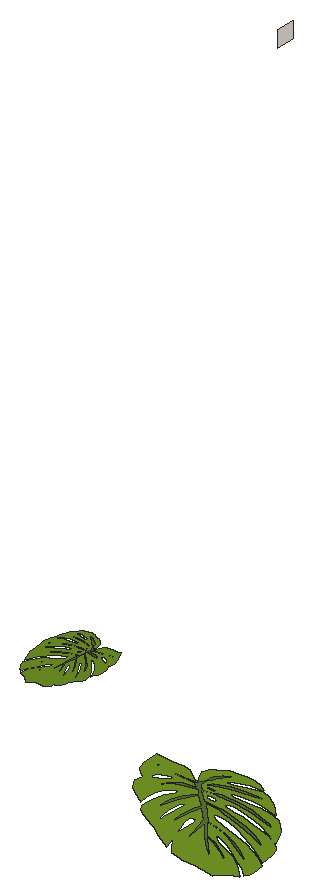
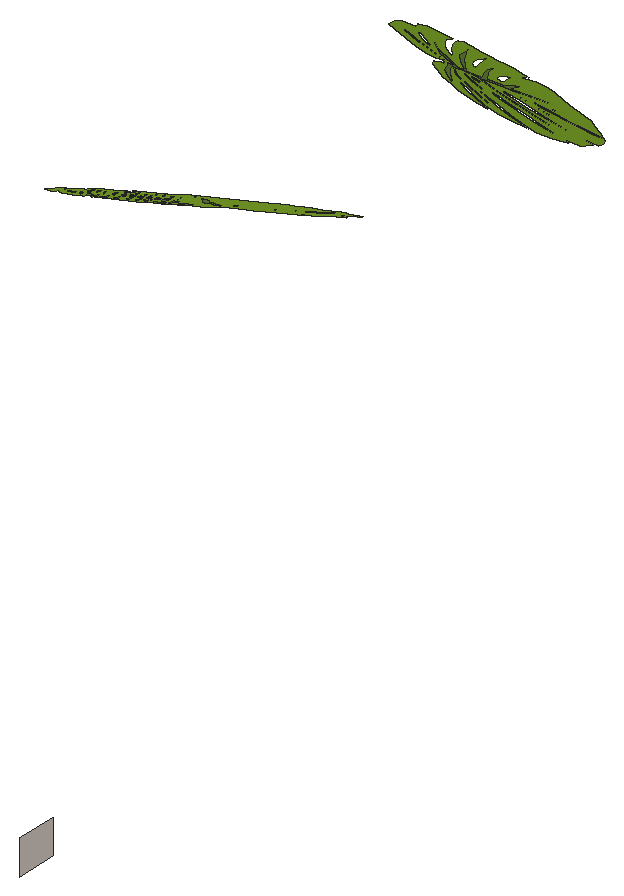
# SketchUp Ruby script. Lengths in inches.
U = 1.inch
M = Sketchup.active_model
def pt(a) = Geom::Point3d.new(a.map { |v| v * U })
def face(e, loops, mat)
  f = e.add_face(loops[0].map { |a| pt(a) })
  loops[1..].each { |l| e.add_face(l.map { |a| pt(a) }).erase! }
  f.material = f.back_material = mat if mat
  f
end
# faces: each face lists its corners as indices into pts; further lists are holes
def faces(e, pts, list, mat = nil) = list.each { |f| face(e, (f[0].is_a?(Array) ? f : [f]).map { |l| l.map { |i| pts[i] } }, mat) }
# xy, xz, yz: faces in a plane at the given z, y or x. An outline is a flat list of corners, or four numbers for a rectangle; further outlines are holes
def ring(l) = l.size == 4 ? [[l[0], l[1]], [l[2], l[1]], [l[2], l[3]], [l[0], l[3]]] : l.each_slice(2).to_a
def flat(e, list, mat, &to3) = list.each { |f| face(e, (f[0].is_a?(Array) ? f : [f]).map { |l| ring(l).map { |u, v| to3.(u, v) } }, mat) }
def xy(e, z, list, mat = nil) = flat(e, list, mat) { |x, y| [x, y, z] }
def xz(e, y, list, mat = nil) = flat(e, list, mat) { |x, z| [x, y, z] }
def yz(e, x, list, mat = nil) = flat(e, list, mat) { |y, z| [x, y, z] }
def lines(e, pts, list) = list.each { |a, b| e.add_line(pt(pts[a]), pt(pts[b])) }
# prism: a flat outline (further loops are holes) pulled along v
def prism(e, loops, v, mat = nil)
  f = face(e, loops, mat); d = Geom::Vector3d.new(v.map { |x| x * U })
  f.pushpull(f.normal.samedirection?(d) ? d.length : -d.length)
end
def box(e, o, s, mat = nil) = prism(e, [[o, [o[0] + s[0], o[1], o[2]], [o[0] + s[0], o[1] + s[1], o[2]], [o[0], o[1] + s[1], o[2]]]], [0, 0, s[2]], mat)
def at(x, y, z, deg = 0) = Geom::Transformation.translation(pt([x, y, z])) * Geom::Transformation.rotation(ORIGIN, Z_AXIS, deg.degrees)
def axes(o, x, y, z) = Geom::Transformation.new([*x, 0, *y, 0, *z, 0, *pt(o).to_a, 1])
def part(name) = M.definitions.add(name)
# library, detail: a bought-in or finely detailed component or shape, given as its bounding box
def library(name, o, s) = part(name).tap { |d| box(d.entities, o, s) }
def detail(e, o, s) = box(e.add_group.entities, o, s)
def put(e, d, t, mat = nil) = e.add_instance(d, t).tap { |i| i.material = mat if mat }
def group(e, t, mat = nil) = e.add_group.tap { |g| g.transformation = t; g.material = mat if mat }.entities
root = M.entities
M.materials.add("[0009_Linen]").color = [250, 240, 230]
M.materials.add("[0059_DarkOliveGreen]").color = [85, 107, 47]
M.materials.add("[0061_OliveDrab]").color = [107, 142, 35]
yz(root,328.15,[[300.43,52.25,304.24,55.45]],"[0009_Linen]")
p = [[413.85,165,15.87],[412.66,164.86,16.11],[411.93,162.875,15.41],[411.97,161.6875,14.86],[412.59,161,14.39],[413.3,160.66,14.0625],
  [412.59,159.58,13.75],[413.01,158.58,13.2],[413.77,158.02,12.75],[415.21,157.53,12.16],[415.68,157.3,11.9375],[415.78,158.5,12.45],
  [416.43,159.72,12.83],[417.45,160.89,13.1],[418.7,161.74,13.15],[419.1,161.9,13.125],[419.24,161.84,13.06],[419.08,161.55,12.97],
  [417.8,160.16,12.68],[416.96,158.93,12.34],[416.26,157.61,11.93],[416.06,156.91,11.67],[416.37,156.3,11.3125],[417.08,155.97,10.98],
  [418.26,155.62,10.52],[419.35,155.32,10.11],[419.91,155.17,9.9],[420.84,154.625,9.41],[421.91,154.24,8.96],[423.01,154.01,8.57],
  [423.59,153.85,8.36],[423.5,154.52,8.68],[423.4,155.52,9.16],[424.51,153.73,8.0625],[424.8125,153.51,7.89],[425.83,153.45,7.6],
  [426.85,153.39,7.31],[429.17,153.85,6.92],[432.48,154.08,6.17],[433.8125,155.1875,6.32],[435.15,155.97,6.33],[436.01,156.4,6.3],
  [434.34,157.54,7.24],[433.04,158.16,7.86],[431.18,158.59,8.53],[429.86,158.85,8.99],[429.22,159.16,9.29],[428.7,159.41,9.53],
  [428.7,159.58,9.61],[429.05,159.63,9.54],[430.09,159.5,9.22],[430.97,159.28,8.89],[432.78,158.59,8.12],[434.29,157.96,7.44],
  [435.26,157.62,7.04],[435.89,157.21,6.7],[436.35,156.78,6.38],[437.04,157.45,6.51],[437.36,158.02,6.68],[437.53,158.54,6.87],
  [437.6,158.94,7.03],[437.78,159.42,7.2],[436.29,160.31,7.98],[434.875,160.78,8.56],[433.64,161,8.98],[431.33,161.24,9.68],
  [429.57,161.3125,10.16],[428.09,161.42,10.59],[426.98,161.5625,10.94],[426.45,161.81,11.19],[426.42,162.15,11.35],[427.25,162.3,11.2],
  [428.39,162.39,10.95],[430.39,162.22,10.36],[432.54,161.79,9.62],[434.92,161.12,8.7],[437.6,160.09,7.55],[437.9,161.81,8.24],
  [437.9375,162.83,8.69],[437.51,163.27,9],[436.53,163.74,9.46],[435.33,164.01,9.89],[433.71,164.12,10.36],[432.33,164.19,10.75],
  [430.29,164.28,11.3125],[428.78,164.22,11.67],[427.6,164.17,11.95],[427.03,164.11,12.07],[426.7,164.26,12.23],[427.05,164.5,12.25],
  [427.92,164.81,12.16],[429.29,164.95,11.87],[432.06,164.83,11.1],[433.6875,164.64,10.6],[435.14,164.38,10.11],[435.81,164.14,9.83],
  [437.14,163.74,9.31],[437.19,164.03,9.42],[436.87,165.02,9.95],[436.52,165.9,10.4375],[435.17,166.9,11.23],[433.76,167.09,11.68],
  [431.5,166.95,12.2],[429.51,166.53,12.52],[427.69,166.23,12.85],[426.9,166.07,12.99],[426.45,166.1,13.12],[426.5,166.28,13.18],
  [427.42,166.65,13.11],[429.64,167.18,12.78],[431.45,167.33,12.38],[434.32,167.32,11.64],[432.88,168.51,12.54],[431.41,169.13,13.2],
  [430.1875,169.24,13.5625],[429.55,169.04,13.64],[427.65,168.38,13.83],[426.23,167.77,13.92],[425.12,167.39,14.04],[424.68,167.35,14.13],
  [424.54,167.51,14.24],[424.78,167.68,14.25],[426.56,168.48,14.16],[427.99,168.93,13.99],[429.26,169.23,13.8],[430.22,169.43,13.64],
  [429.04,169.87,14.14],[427.93,170,14.49],[426.5,169.8125,14.77],[425.16,169.43,14.94],[423.79,169.16,15.17],[423.08,168.68,15.14],
  [421.9,168.09,15.18],[420.89,167.41,15.14],[420.4,166.5,14.85],[420.55,165.56,14.39],[420.89,165.01,14.06],[420.2,164.81,14.14],
  [419.625,165.26,14.5],[418.65,165.72,14.95],[417.39,165.69,15.27],[415.54,165.35,15.59],[417.35,163.83,14.44],[413.875,163.56,15.21],
  [416.11,163.94,14.8125],[420.77,164.75,13.97],[421.34,165.45,14.14],[422.24,166.95,14.58],[423.42,167.88,14.7],[424.45,168.43,14.68],
  [422.86,166.86,14.38],[421.93,165.56,14.04],[421.63,164.83,13.79],[422.94,165.99,13.97],[425.51,167.09,13.8],[427.57,167.66,13.53],
  [429.69,168.11,13.1875],[430.76,168.25,12.97],[427.48,167.34,13.41],[425.53,166.7,13.625],[423.38,165.83,13.79],[422.26,165.08,13.74],
  [421.8,164.66,13.66],[421.92,164.39,13.52],[422.27,164.34,13.4],[423.22,164.59,13.27],[424.17,165,13.21],[425.3,165.27,13.04],
  [428.57,165.79,12.43],[430.65,165.95,11.97],[432.61,165.8,11.4],[434.19,165.7,10.95],[434.79,165.42,10.66],[431.74,165.625,11.54],
  [430.01,165.56,11.96],[427.28,165.27,12.53],[424.87,164.77,12.93],[422.24,164.1,13.3],[423.61,163.03,12.47],[425.64,163.29,12.06],
  [427.5625,163.49,11.66],[431.54,163.29,10.55],[433.51,162.92,9.87],[434.83,162.59,9.39],[435.44,162.3,9.1],[433.58,162.65,9.73],
  [430.51,162.96,10.66],[426.58,163.0625,11.72],[424.22,162.74,12.18],[426.33,160.69,10.72],[427.91,160.84,10.38],[429.85,160.64,9.79],
  [431.71,160.18,9.11],[433.11,159.7,8.53],[434.65,158.97,7.81],[431.46,160,9.09],[429.62,160.42,9.75],[427.9,160.56,10.26],
  [426.35,160.45,10.61],[427.6875,158.86,9.55],[429.39,158.57,8.98],[430.92,158.08,8.37],[432.17,157.48,7.78],[432.72,156.9,7.375],
  [430.625,157.9,8.36],[429.06,158.3,8.94],[427.8,158.53,9.37],[429.09,157.29,8.48],[429.77,156.63,8.01],[430.74,155.78,7.38],
  [430.57,155.89,7.48],[428.69,157.14,8.52],[427.2,158.4,9.47],[426.0625,159.92,10.44],[425.3,156.34,9.03],[425.31,160.42,10.86],
  [423.96,161.63,11.75],[422.75,159.88,11.28],[421.51,157.05,10.33],[421.95,159.13,11.15],[422.87,161.0625,11.78],[423.61,162.08,12.04],
  [422.29,163.09,12.83],[420.16,160.89,12.4],[418.05,157.68,11.5],[418.92,160.25,12.43],[420.4,161.95,12.8125],[422.03,163.4,13.04],
  [421.59,163.82,13.34],[419.95,163.24,13.51],[417.77,162.48,13.73],[415.57,160.74,13.51],[417.07,162.3,13.83],[418.79,163.47,13.9],
  [420.73,163.92,13.61],[421.05,164.13,13.62],[420.41,164.43,13.92],[420.16,159.31,11.6875],[420.89,160.49,12.03],[421.27,160.78,12.0625],
  [421.54,160.85,12.02],[421.65,160.71,11.93],[421.43,160.24,11.78],[420.9,159.11,11.41],[420.33,157.87,11],[419.89,156.5625,10.53],
  [419.66,155.95,10.31],[419.72,157.81,11.125],[423.55,159.45,10.88],[423.89,159.875,10.98],[424.29,159.9,10.89],[424.5,159.71,10.75],
  [424.54,159.3,10.56],[424.4,158.97,10.44],[423.89,157.66,9.99],[423.4,156.44,9.57],[423.33,158.3,10.42],[414.96,162.42,14.42],
  [415.93,162.94,14.4],[416.79,163.24,14.32],[417.25,163.21,14.1875],[417.4,163.07,14.09],[415.97,162.18,14.06],[414.7,161.48,14.07],
  [414.33,161.35,14.1],[414.36,161.85,14.32],[423.95,164.2,12.91],[424.6875,164.24,12.74],[425.24,164.08,12.52],[425.1875,163.86,12.4375],
  [424.48,163.625,12.51],[423.63,163.68,12.75],[423.36,163.9375,12.94],[422.67,165.07,13.63],[423.43,165.26,13.51],[424,165.26,13.37],
  [423.98,165.04,13.27],[423.15,164.84,13.4],[422.55,164.82,13.55],[406.4375,162.9,32.91],[407.23,162.8,33.07],[407.7,161.5,32.61],
  [407.68,160.71,32.25],[407.27,160.26,31.94],[406.81,160.03,31.72],[407.27,159.32,31.52],[406.99,158.66,31.15],[406.49,158.29,30.86],
  [405.54,157.96,30.47],[405.23,157.82,30.32],[405.17,158.6,30.66],[404.74,159.41,30.91],[404.07,160.19,31.08],[403.24,160.75,31.12],
  [402.97,160.85,31.1],[402.88,160.81,31.06],[402.99,160.62,31],[403.84,159.7,30.81],[404.39,158.89,30.59],[404.85,158.02,30.3125],
  [404.98,157.56,30.14],[404.78,157.16,29.91],[404.31,156.9375,29.69],[403.53,156.7,29.38],[402.81,156.51,29.11],[402.44,156.41,28.97],
  [401.83,156.05,28.65],[401.12,155.79,28.36],[400.4,155.64,28.1],[400.01,155.54,27.96],[400.07,155.98,28.17],[400.14,156.64,28.48],
  [399.41,155.46,27.76],[399.2,155.32,27.65],[398.53,155.27,27.46],[397.86,155.23,27.27],[396.33,155.54,27.01],[394.14,155.6875,26.51],
  [393.26,156.42,26.62],[392.38,156.93,26.62],[391.82,157.22,26.6],[392.91,157.97,27.22],[393.77,158.38,27.625],[395,158.66,28.07],
  [395.87,158.84,28.37],[396.29,159.04,28.57],[396.64,159.21,28.73],[396.64,159.32,28.78],[396.41,159.35,28.74],[395.72,159.27,28.53],
  [395.14,159.125,28.3125],[393.95,158.67,27.8],[392.95,158.25,27.35],[392.3125,158.02,27.09],[391.9,157.75,26.86],[391.59,157.47,26.65],
  [391.14,157.91,26.74],[390.93,158.29,26.85],[390.8125,158.63,26.98],[390.76,158.9,27.08],[390.65,159.22,27.2],[391.63,159.8,27.71],
  [392.5625,160.11,28.09],[393.38,160.25,28.36],[394.9,160.42,28.83],[396.0625,160.46,29.15],[397.04,160.53,29.43],[397.78,160.63,29.66],
  [398.125,160.79,29.83],[398.15,161.02,29.93],[397.6,161.11,29.84],[396.84,161.17,29.67],[395.52,161.06,29.28],[394.11,160.78,28.79],
  [392.54,160.33,28.18],[390.77,159.65,27.42],[390.57,160.79,27.88],[390.54,161.46,28.18],[390.82,161.76,28.38],[391.47,162.07,28.6875],
  [392.26,162.24,28.97],[393.33,162.3125,29.28],[394.24,162.36,29.53],[395.59,162.42,29.91],[396.59,162.38,30.15],[397.36,162.35,30.33],
  [397.74,162.31,30.41],[397.96,162.41,30.51],[397.73,162.57,30.52],[397.16,162.77,30.46],[396.25,162.87,30.28],[394.42,162.78,29.77],
  [393.35,162.66,29.43],[392.39,162.49,29.11],[391.95,162.33,28.93],[391.07,162.07,28.58],[391.03,162.25,28.66],[391.25,162.91,29.01],
  [391.48,163.49,29.33],[392.37,164.15,29.85],[393.3,164.28,30.15],[394.79,164.18,30.49],[396.1,163.91,30.71],[397.3,163.71,30.92],
  [397.83,163.6,31.01],[398.125,163.62,31.1],[398.09,163.74,31.14],[397.48,163.99,31.1],[396.02,164.33,30.875],[394.83,164.43,30.61],
  [392.93,164.43,30.12],[393.88,165.21,30.72],[394.85,165.625,31.15],[395.66,165.69,31.39],[396.08,165.5625,31.44],[397.33,165.125,31.57],
  [398.27,164.73,31.63],[399,164.47,31.71],[399.29,164.45,31.77],[399.39,164.55,31.84],[399.23,164.66,31.85],[398.05,165.19,31.78],
  [397.11,165.49,31.68],[396.27,165.6875,31.55],[395.63,165.82,31.44],[396.42,166.11,31.77],[397.15,166.2,32],[398.09,166.07,32.1875],
  [398.98,165.82,32.3],[399.88,165.64,32.46],[400.35,165.32,32.43],[401.13,164.9375,32.46],[401.8,164.49,32.43],[402.11,163.89,32.24],
  [402.02,163.27,31.94],[401.79,162.9,31.72],[402.25,162.77,31.78],[402.63,163.07,32.01],[403.27,163.375,32.3125],[404.11,163.35,32.52],
  [405.32,163.125,32.73],[404.13,162.125,31.97],[406.42,161.95,32.48],[404.95,162.2,32.22],[401.875,162.73,31.66],[401.5,163.19,31.77],
  [400.9,164.18,32.0625],[400.12,164.8,32.14],[399.45,165.16,32.125],[400.5,164.12,31.93],[401.11,163.26,31.71],[401.3,162.78,31.54],
  [400.44,163.55,31.66],[398.74,164.27,31.55],[397.38,164.66,31.37],[395.98,164.95,31.14],[395.28,165.04,31],[397.45,164.44,31.29],
  [398.73,164.02,31.43],[400.15,163.45,31.54],[400.89,162.95,31.51],[401.19,162.67,31.46],[401.12,162.5,31.36],[400.88,162.46,31.29],
  [400.26,162.625,31.2],[399.625,162.89,31.16],[398.88,163.07,31.05],[396.73,163.42,30.65],[395.35,163.53,30.34],[394.06,163.43,29.96],
  [393.01,163.36,29.67],[392.62,163.17,29.48],[394.64,163.31,30.06],[395.78,163.27,30.33],[397.58,163.07,30.71],[399.17,162.75,30.97],
  [400.91,162.3,31.22],[400,161.6,30.67],[398.66,161.76,30.4],[397.39,161.9,30.14],[394.76,161.77,29.4],[393.46,161.52,28.96],
  [392.6,161.31,28.64],[392.1875,161.11,28.44],[393.42,161.35,28.87],[395.45,161.55,29.48],[398.04,161.62,30.18],[399.59,161.4,30.48],
  [398.2,160.05,29.52],[397.16,160.15,29.29],[395.88,160.02,28.9],[394.65,159.72,28.45],[393.73,159.4,28.07],[392.72,158.92,27.59],
  [394.82,159.6,28.44],[396.03,159.875,28.88],[397.17,159.97,29.21],[398.19,159.9,29.44],[397.31,158.84,28.74],[396.18,158.65,28.37],
  [395.18,158.33,27.96],[394.35,157.9375,27.57],[393.99,157.55,27.31],[395.37,158.21,27.96],[396.4,158.47,28.34],[397.23,158.625,28.625],
  [396.38,157.81,28.04],[395.93,157.37,27.73],[395.29,156.8125,27.3125],[395.4,156.89,27.375],[396.65,157.71,28.0625],[397.63,158.54,28.69],
  [398.38,159.54,29.33],[398.89,157.18,28.4],[398.88,159.87,29.61],[399.77,160.67,30.2],[400.57,159.52,29.88],[401.39,157.65,29.26],
  [401.09,159.02,29.8],[400.49,160.3,30.21],[400,160.97,30.39],[400.87,161.64,30.91],[402.28,160.18,30.62],[403.67,158.06,30.03],
  [403.1,159.76,30.64],[402.12,160.89,30.9],[401.04,161.84,31.05],[401.33,162.12,31.25],[402.41,161.74,31.36],[403.85,161.23,31.5],
  [405.3,160.09,31.36],[404.3125,161.12,31.57],[403.18,161.88,31.62],[401.9,162.18,31.42],[401.69,162.32,31.43],[402.11,162.52,31.63],
  [402.28,159.14,30.15],[401.8,159.92,30.38],[401.54,160.11,30.4],[401.37,160.16,30.375],[401.29,160.07,30.32],[401.4375,159.75,30.21],
  [401.79,159.01,29.97],[402.16,158.19,29.7],[402.46,157.33,29.39],[402.61,156.92,29.24],[402.5625,158.15,29.78],[400.04,159.23,29.62],
  [399.8125,159.51,29.6875],[399.55,159.53,29.63],[399.41,159.41,29.54],[399.39,159.13,29.41],[399.48,158.92,29.33],[399.82,158.05,29.03],
  [400.14,157.25,28.75],[400.1875,158.48,29.32],[405.71,161.19,31.96],[405.0625,161.54,31.95],[404.5,161.73,31.89],[404.2,161.71,31.8],
  [404.1,161.625,31.74],[405.04,161.04,31.72],[405.88,160.57,31.73],[406.125,160.49,31.75],[406.1,160.82,31.89],[399.78,162.37,30.96],
  [399.29,162.4,30.85],[398.92,162.29,30.71],[398.96,162.15,30.65],[399.42,161.99,30.7],[399.98,162.02,30.86],[400.16,162.2,30.98],
  [400.62,162.94,31.43],[400.11,163.06,31.36],[399.74,163.07,31.27],[399.76,162.92,31.2],[400.3,162.79,31.29],[400.7,162.78,31.38]]
faces(root,p,[[[0,1,2,3,4,5,6,7,8,9,10,11,12,13,14,15,16,17,18,19,20,21,22,23,24,25,26,27,28,29,30,31,32,33,34,35,36,37,38,39,40,41,42,43,44,45,46,47,48,49,50,51,52,53,54,55,56,57,58,59,60,61,62,63,64,65,66,67,68,69,70,71,72,73,74,75,76,77,78,79,80,81,82,83,84,85,86,87,88,89,90,91,92,93,94,95,80,96,97,98,99,100,101,102,103,104,105,106,107,108,109,110,111,112,113,114,115,116,117,118,119,120,121,122,123,124,125,126,127,128,129,130,131,132,133,134,135,136,137,138,139,140,141],[142,143,144,145,146,147,148,149,150,151,152,153,154,155,156,157,158,159,160,161,162,163,164,165,166,167,168,169,170,171,172,173,174,175,176,177,178,179,180,181,182,183,184,185,186,187,188,189,190,191,192,193,194,195,196,197,198,199,200,201,202,203,204,205,206,207,208,209,210,211,212,213,214,215,216,217,218,219,220,221,222,223,224,225,226,227,228,229,230,231,232,233,234,235,236],[237,238,239,240,241,242,243,244,245,246,247],[248,249,250,251,252,253,254,255,256],[257,258,259,260,261,262,263,264,265],[266,267,268,269,270,271,272],[273,274,275,276,277,278]],[[279,280,281,282,283,284,285,286,287,288,289,290,291,292,293,294,295,296,297,298,299,300,301,302,303,304,305,306,307,308,309,310,311,312,313,314,315,316,317,318,319,320,321,322,323,324,325,326,327,328,329,330,331,332,333,334,335,336,337,338,339,340,341,342,343,344,345,346,347,348,349,350,351,352,353,354,355,356,357,358,359,360,361,362,363,364,365,366,367,368,369,370,371,372,373,374,359,375,376,377,378,379,380,381,382,383,384,385,386,387,388,389,390,391,392,393,394,395,396,397,398,399,400,401,402,403,404,405,406,407,408,409,410,411,412,413,414,415,416,417,418,419,420],[421,422,423,424,425,426,427,428,429,430,431,432,433,434,435,436,437,438,439,440,441,442,443,444,445,446,447,448,449,450,451,452,453,454,455,456,457,458,459,460,461,462,463,464,465,466,467,468,469,470,471,472,473,474,475,476,477,478,479,480,481,482,483,484,485,486,487,488,489,490,491,492,493,494,495,496,497,498,499,500,501,502,503,504,505,506,507,508,509,510,511,512,513,514,515],[516,517,518,519,520,521,522,523,524,525,526],[527,528,529,530,531,532,533,534,535],[536,537,538,539,540,541,542,543,544],[545,546,547,548,549,550,551],[552,553,554,555,556,557]]],"[0061_OliveDrab]")
faces(root,p,[[143,142,236,235,234,233,232,231,230,229,228,227,226,225,224,223,222,221,220,219,218,217,216,215,214,213,212,211,210,209,208,207,206,205,204,203,202,201,200,199,198,197,196,195,194,193,192,191,190,189,188,187,186,185,184,183,182,181,180,179,178,177,176,175,174,173,172,171,170,169,168,167,166,165,164,163,162,161,160,159,158,157,156,155,154,153,152,151,150,149,148,147,146,145,144],[422,421,515,514,513,512,511,510,509,508,507,506,505,504,503,502,501,500,499,498,497,496,495,494,493,492,491,490,489,488,487,486,485,484,483,482,481,480,479,478,477,476,475,474,473,472,471,470,469,468,467,466,465,464,463,462,461,460,459,458,457,456,455,454,453,452,451,450,449,448,447,446,445,444,443,442,441,440,439,438,437,436,435,434,433,432,431,430,429,428,427,426,425,424,423]],"[0059_DarkOliveGreen]")
